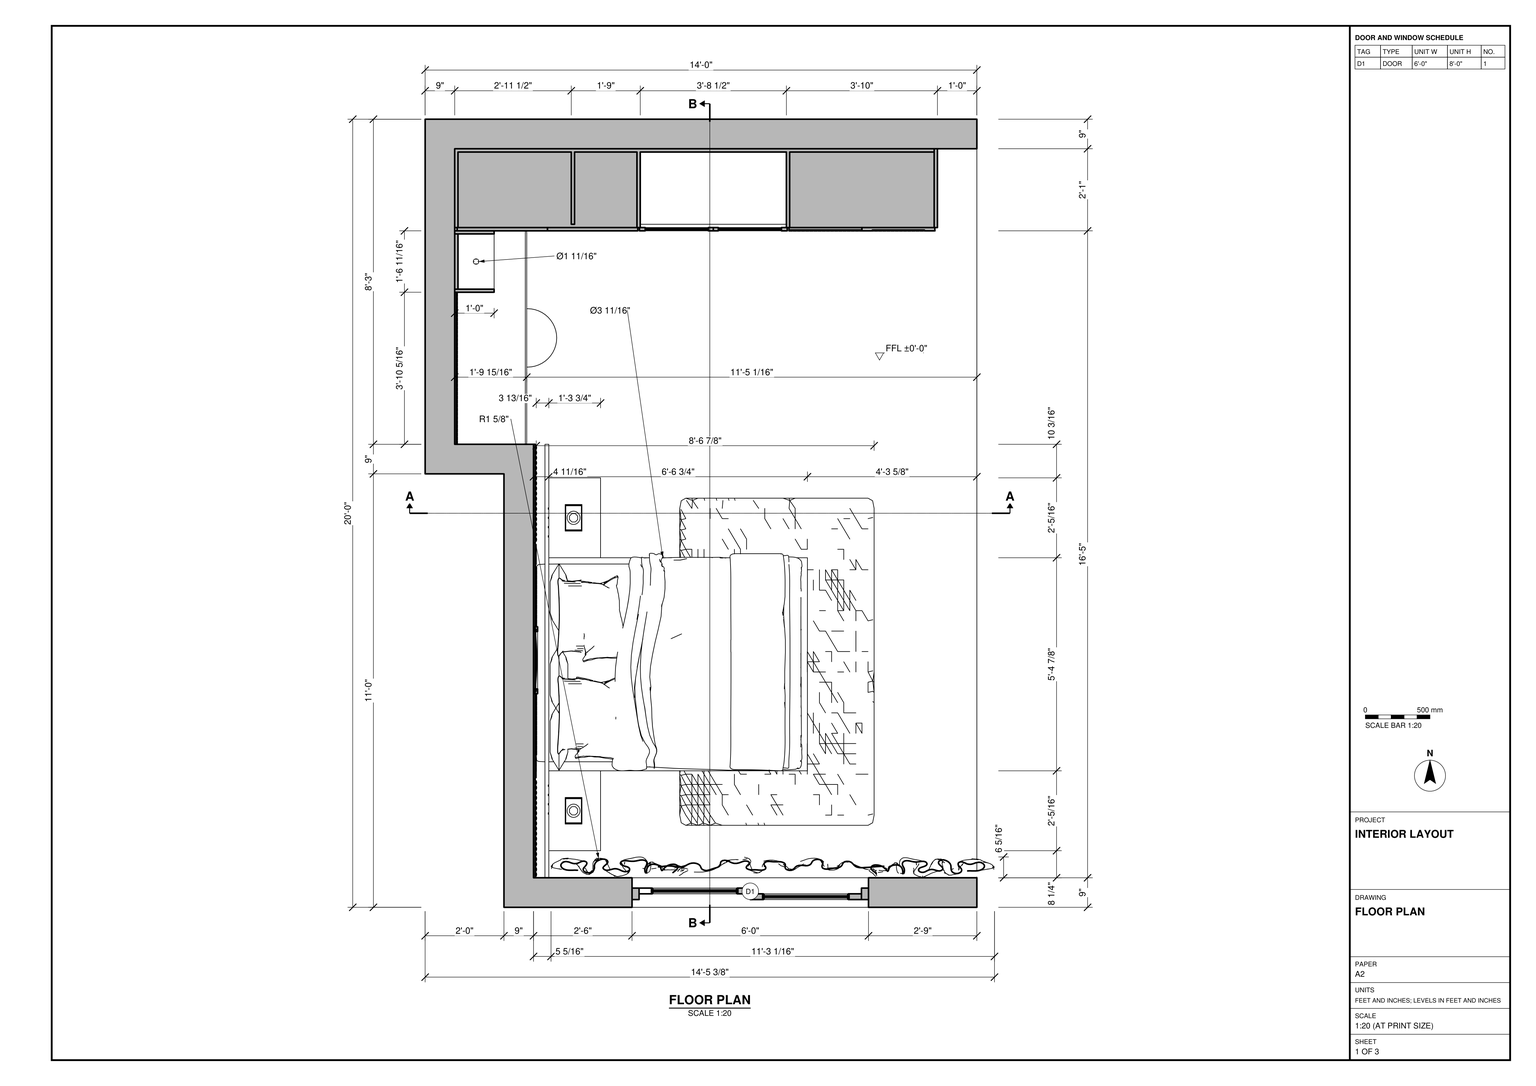
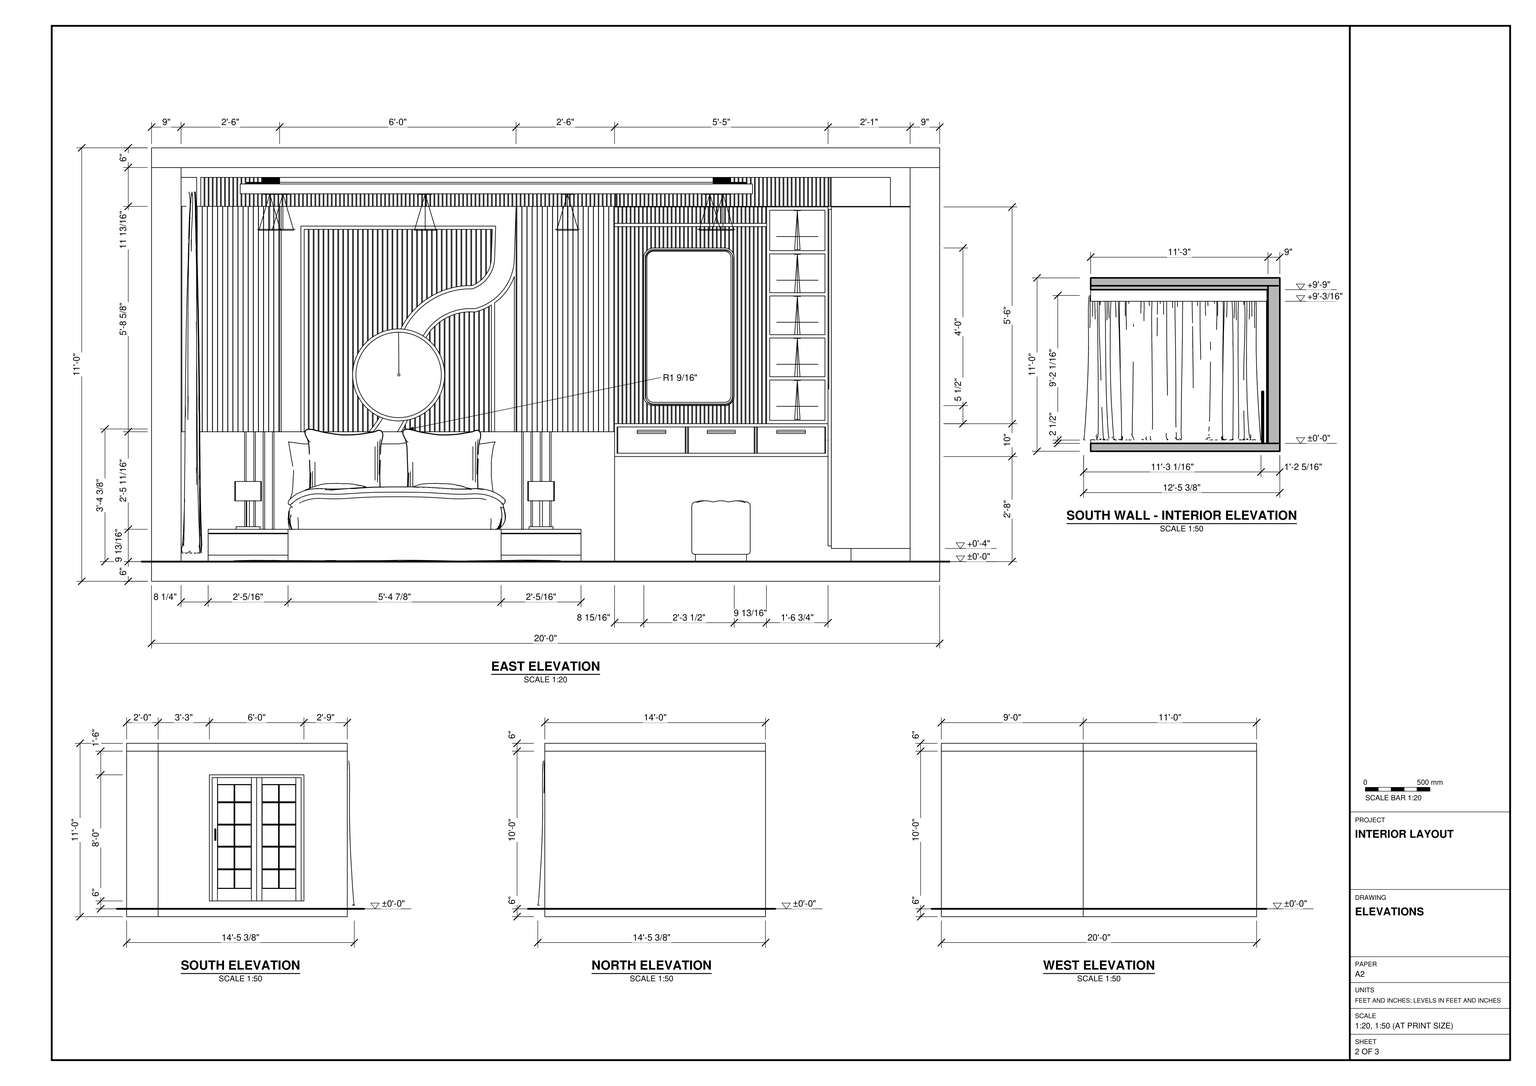
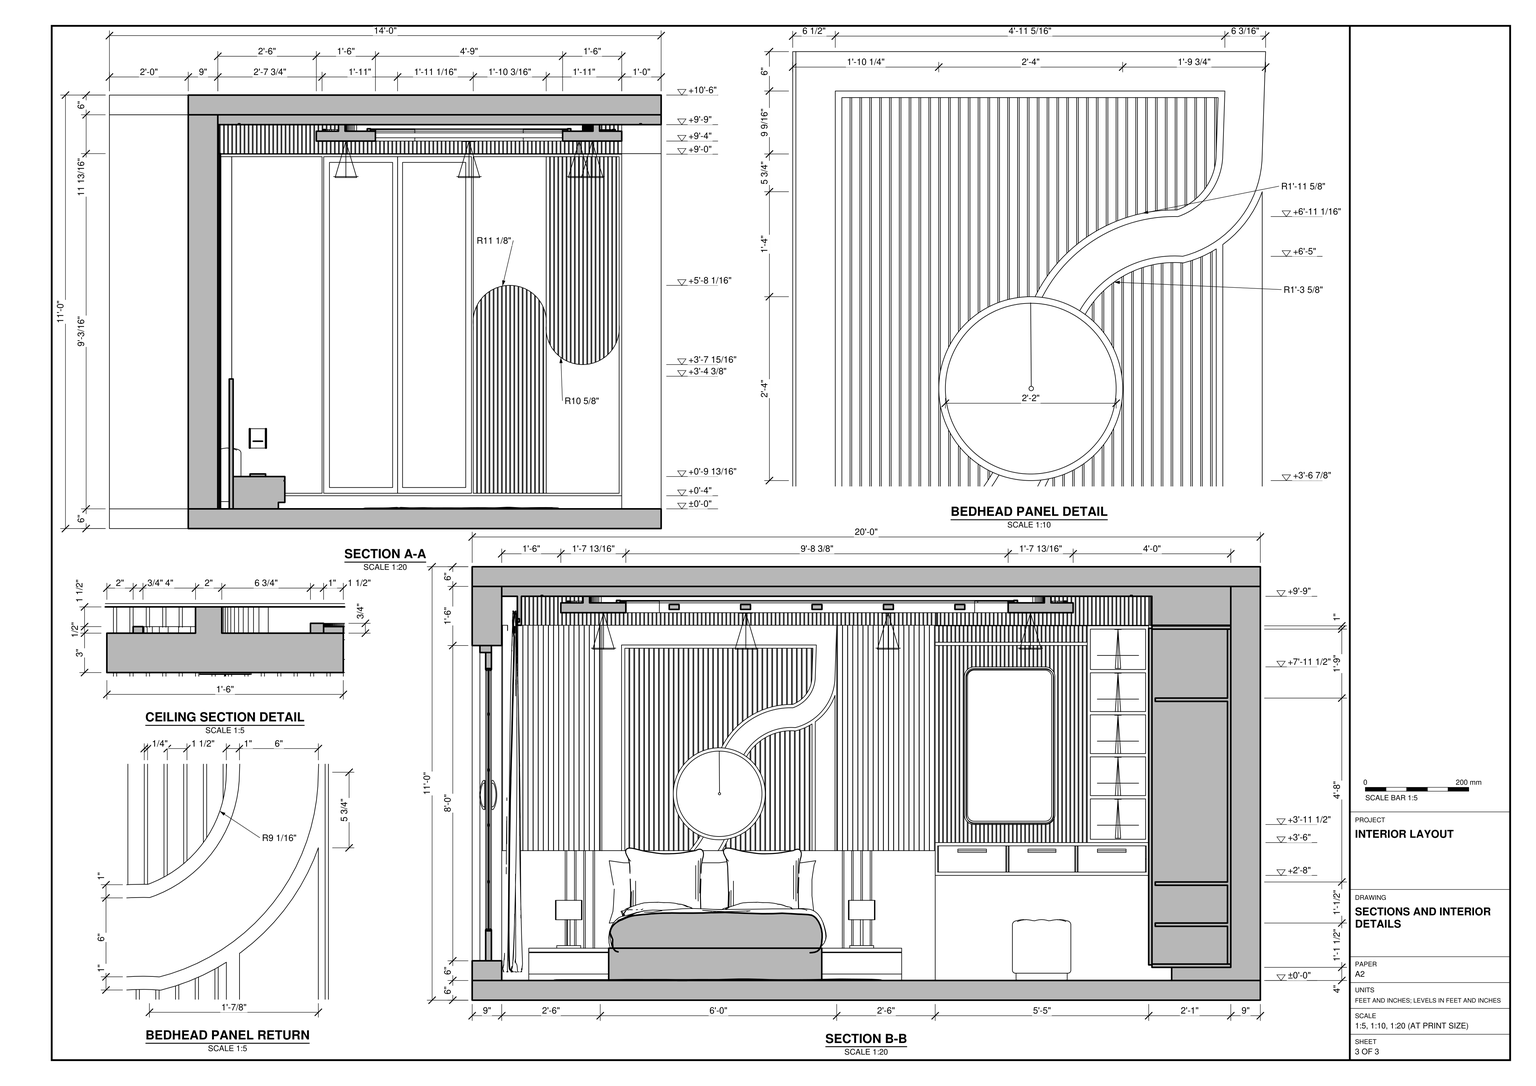
Build the bedroom interior in SketchUp from task_files/diagram_01.pdf. Work in feet and inches. The finished model measures 14'-5 3/8" east to west, 20'-0" north to south and 11'-0" high, with one finished floor level at ±0'-0". Follow the stepped west wall in plan and leave the east side open as drawn. Model the 9" walls, the floor and overhead slabs, and the glazed sliding door in the south wall. Use the sections to set out the ceiling detail above the bed and dressing area.

Place the bed with its head against the inset length of the west wall and a low bedside unit on each side. Follow the enlarged detail for the vertical ribs, circular centre and curved band of the bedhead panel. Fit the dressing counter, drawers, mirror, side shelving and stool into the wider part of the room. Continue the storage along the north wall, matching the panel divisions and curved ribbed fronts in section. Include the curtain at the south door and the rug extending beyond the foot of the bed. Decor and loose items may be any suitable library components placed as shown.

Keep the walls and slabs in separate groups or components, group each furniture or joinery piece separately, and use components for repeated parts. Save one SketchUp model as output_files/bedroom_with_a_stepped_plan_and_built_in_dressing_area.skp.

# SketchUp Ruby script. Lengths in inches.
U = 1.inch
M = Sketchup.active_model
def pt(a) = Geom::Point3d.new(a.map { |v| v * U })
def face(e, loops, mat)
  f = e.add_face(loops[0].map { |a| pt(a) })
  loops[1..].each { |l| e.add_face(l.map { |a| pt(a) }).erase! }
  f.material = f.back_material = mat if mat
  f
end
# faces: each face lists its corners as indices into pts; further lists are holes
def faces(e, pts, list, mat = nil) = list.each { |f| face(e, (f[0].is_a?(Array) ? f : [f]).map { |l| l.map { |i| pts[i] } }, mat) }
# xy, xz, yz: faces in a plane at the given z, y or x. An outline is a flat list of corners, or four numbers for a rectangle; further outlines are holes
def ring(l) = l.size == 4 ? [[l[0], l[1]], [l[2], l[1]], [l[2], l[3]], [l[0], l[3]]] : l.each_slice(2).to_a
def flat(e, list, mat, &to3) = list.each { |f| face(e, (f[0].is_a?(Array) ? f : [f]).map { |l| ring(l).map { |u, v| to3.(u, v) } }, mat) }
def xy(e, z, list, mat = nil) = flat(e, list, mat) { |x, y| [x, y, z] }
def xz(e, y, list, mat = nil) = flat(e, list, mat) { |x, z| [x, y, z] }
def yz(e, x, list, mat = nil) = flat(e, list, mat) { |y, z| [x, y, z] }
def lines(e, pts, list) = list.each { |a, b| e.add_line(pt(pts[a]), pt(pts[b])) }
# prism: a flat outline (further loops are holes) pulled along v
def prism(e, loops, v, mat = nil)
  f = face(e, loops, mat); d = Geom::Vector3d.new(v.map { |x| x * U })
  f.pushpull(f.normal.samedirection?(d) ? d.length : -d.length)
end
def box(e, o, s, mat = nil) = prism(e, [[o, [o[0] + s[0], o[1], o[2]], [o[0] + s[0], o[1] + s[1], o[2]], [o[0], o[1] + s[1], o[2]]]], [0, 0, s[2]], mat)
def at(x, y, z, deg = 0) = Geom::Transformation.translation(pt([x, y, z])) * Geom::Transformation.rotation(ORIGIN, Z_AXIS, deg.degrees)
def axes(o, x, y, z) = Geom::Transformation.new([*x, 0, *y, 0, *z, 0, *pt(o).to_a, 1])
def part(name) = M.definitions.add(name)
# library, detail: a bought-in or finely detailed component or shape, given as its bounding box
def library(name, o, s) = part(name).tap { |d| box(d.entities, o, s) }
def detail(e, o, s) = box(e.add_group.entities, o, s)
def put(e, d, t, mat = nil) = e.add_instance(d, t).tap { |i| i.material = mat if mat }
def group(e, t, mat = nil) = e.add_group.tap { |g| g.transformation = t; g.material = mat if mat }.entities
root = M.entities
M.materials.add("0993 AP 7924 MOON YEAR").color = [247, 236, 211]
M.materials.add("False ceiling Light").color = [250, 225, 158]
M.materials.add("Teddy_Skin").color = [228, 212, 199]
M.materials.add("[Color_A11]").color = [255, 247, 241]
M.materials.add("[Wood Veneer 01]2").color = [66, 44, 30]
M.materials.add("[Wood Veneer 01]3").color = [120, 70, 37]
c1 = library("Group5_1",[-7.56,-66.38,0.11],[6.33,135.04,120.95])
c2 = library("1",[0,-0.85,0],[30,0.85,108.17])
c3 = library("sliding door",[152.33,87.51,0.76],[72,5.24,96])
c4 = library("Vanity Chair",[-7.875,-7.875,0],[15.75,15.75,16.41])
c5 = library("Group\#4",[0,-1.41,0],[72,1.41,108.17])
c6 = library("Group\#11",[0,-21.9375,2],[66,21.9375,76])
c7 = library("Group\#17",[-25,0,0],[25,147,104])
c8 = library("Group\#10",[0,0,-5.36],[198,135,41.44])
c9 = library("Group\#26",[0,0,-14.11],[156,93,16.11])
c10 = part("Group155\#1")
box(c10.entities,[-9.125,-4.41,0],[1,8.82,0.25])
c11 = part("Group156\#1")
box(c11.entities,[-7.875,-4.41,0],[1,8.82,0.25])
c12 = part("Group157\#1")
box(c12.entities,[-6.625,-4.41,0],[1,8.82,0.25])
c13 = part("Group158\#1")
box(c13.entities,[-5.375,-4.41,0],[1,8.82,0.25])
c14 = part("Group159\#1")
box(c14.entities,[-4.125,-4.41,0],[1,8.82,0.25])
c15 = part("Group160\#1")
box(c15.entities,[-2.875,-4.41,0],[1,8.82,0.25])
c16 = part("Group161\#1")
box(c16.entities,[-1.625,-4.41,0],[1,8.82,0.25])
c17 = part("Group162\#1")
box(c17.entities,[-0.375,-4.41,0],[1,8.82,0.25])
c18 = part("Group163\#1")
box(c18.entities,[0.875,-4.41,0],[1,8.82,0.25])
c19 = part("Group164\#1")
box(c19.entities,[2.125,-4.41,0],[1,8.82,0.25])
c20 = part("Group165\#1")
box(c20.entities,[3.375,-4.41,0],[1,8.82,0.25])
c21 = part("Group166\#1")
box(c21.entities,[4.625,-4.41,0],[1,8.82,0.25])
c22 = part("Group167\#1")
box(c22.entities,[5.875,-4.41,0],[1,8.82,0.25])
c23 = part("Group168\#1")
box(c23.entities,[7.125,-4.41,0],[1,8.82,0.25])
c24 = part("Group169\#1")
xy(c24.entities,0,[[8.375,-4.41,9.125,4.41]])
xy(c24.entities,0.25,[[8.375,-4.41,9.125,4.41]])
yz(c24.entities,8.375,[[-4.41,0,4.41,0.25]])
c25 = part("Group153\#1")
put(c25.entities,c10,at(0,0,0))
put(c25.entities,c11,at(0,0,0))
put(c25.entities,c12,at(0,0,0))
put(c25.entities,c13,at(0,0,0))
put(c25.entities,c14,at(0,0,0))
put(c25.entities,c15,at(0,0,0))
put(c25.entities,c16,at(0,0,0))
put(c25.entities,c17,at(0,0,0))
put(c25.entities,c18,at(0,0,0))
put(c25.entities,c19,at(0,0,0))
put(c25.entities,c20,at(0,0,0))
put(c25.entities,c21,at(0,0,0))
put(c25.entities,c22,at(0,0,0))
put(c25.entities,c23,at(0,0,0))
put(c25.entities,c24,at(0,0,0))
c26 = library("Group169\#2",[-32.74,-4.41,0],[65.48,8.82,0.25])
c27 = library("Group223\#2",[-70.5,-4.41,0],[141,8.82,0.25])
c28 = library("Group337\#2",[-63.25,-4.41,0],[126.75,8.82,0.25])
g1 = group(root,at(168,0,6,90))
put(g1,c1,axes([16.56,61.01,2.42],[1,0,0],[0,1,0],[0,0,0.91]))
g2 = group(g1,at(0,0,0))
xy(g2,0,[[0,0,0,144,141,144,141,135,9,135,9,0],[231,0,231,12,213,12,213,159,132,159,132,168,240,168,240,0],[132,144,141,159]],"0993 AP 7924 MOON YEAR")
xy(g2,4,[[213,12,231,159]],"0993 AP 7924 MOON YEAR")
xy(g2,6,[[0,33,9,105]],"0993 AP 7924 MOON YEAR")
xy(g2,102,[[0,33,9,105]],"0993 AP 7924 MOON YEAR")
xy(g2,120,[[0,0,9,0,9,135,141,135,141,159,231,159,231,0,240,0,240,168,132,168,132,144,0,144]],"0993 AP 7924 MOON YEAR")
xz(g2,0,[[0,0,9,120],[231,0,240,120]],"0993 AP 7924 MOON YEAR")
xz(g2,12,[[213,0,231,4]],"0993 AP 7924 MOON YEAR")
xz(g2,33,[[0,6,9,102]],"0993 AP 7924 MOON YEAR")
xz(g2,105,[[0,6,9,102]],"0993 AP 7924 MOON YEAR")
xz(g2,135,[[9,0,141,120]],"0993 AP 7924 MOON YEAR")
xz(g2,144,[[0,0,132,120]],"0993 AP 7924 MOON YEAR")
xz(g2,159,[[141,0,213,0,213,4,231,4,231,120,141,120]],"0993 AP 7924 MOON YEAR")
xz(g2,168,[[132,0,240,120]],"0993 AP 7924 MOON YEAR")
yz(g2,0,[[[0,0,144,120],[33,6,105,102]]],"0993 AP 7924 MOON YEAR")
yz(g2,9,[[[0,0,135,120],[33,6,105,102]]],"0993 AP 7924 MOON YEAR")
yz(g2,132,[[144,0,168,120]],"0993 AP 7924 MOON YEAR")
yz(g2,141,[[135,0,159,120]],"0993 AP 7924 MOON YEAR")
yz(g2,213,[[12,0,159,4]],"0993 AP 7924 MOON YEAR")
yz(g2,231,[[0,0,0,120,159,120,159,4,12,4,12,0]],"0993 AP 7924 MOON YEAR")
yz(g2,240,[[0,0,168,120]],"0993 AP 7924 MOON YEAR")
# 2 loose lines left out
put(g2,c2,at(9,135,0),"Teddy_Skin")
put(g2,c2,at(111,135,0),"Teddy_Skin")
put(g2,c3,at(-85.25,257.33,5.24,-90))
put(g2,c4,axes([173.4,136.84,0],[1.13,0,0],[0,1.13,0],[0,0,1.13]))
put(g2,c5,at(39,135,0))
put(g2,c6,axes([141,159,30],[0.98485,0,0],[0,1,0],[0,0,1]),"[Color_A11]")
put(g2,c7,at(231,12,4),"[Wood Veneer 01]3")
put(g1,c8,axes([0,0,0],[1.21212,0,0],[0,1.24444,0],[0,0,1.12]))
g3 = group(g1,at(0,0,120))
xy(g3,0,[[0,0,0,144,132,144,132,168,240,168,240,0,231,0,231,159,141,159,141,135,9,135,9,0],[9,0,9,135,141,135,141,159,231,159,231,0]])
xy(g3,6,[[0,0,240,0,240,168,132,168,132,144,0,144]])
xz(g3,0,[[0,0,240,6]])
xz(g3,144,[[0,0,132,6]])
xz(g3,168,[[132,0,240,6]])
yz(g3,0,[[0,0,144,6]])
yz(g3,132,[[144,0,168,6]])
yz(g3,240,[[0,0,168,6]])
g4 = group(g3,at(9,0,0))
xy(g4,-11.83,[[4.75,0,4.75,134.75,5,135,6,135,6,0],[216,0,216,12,197.97,12,197.97,153,132.5,153,132.5,134.75,6,134.75,6,135,132,135,132,159,222,159,222,0]])
xy(g4,-10.83,[[4.75,1,5.375,126]])
xy(g4,-9.83,[[4.75,1,5.375,126]])
xy(g4,-3,[[0,0,0,135,5,135,4.75,134.75,4.75,0],[[6,0,6,134.75,132.5,134.75,132.5,153,197.97,153,197.97,12,216,12,216,0],[12,6,191.97,6,191.97,147,138.5,147,138.5,128.75,12,128.75]],[12.5,6.5,12.5,128.25,139,128.25,139,146.5,191.47,146.5,191.47,6.5]])
xy(g4,-2.75,[[[12,6,12,128.75,138.5,128.75,138.5,147,191.97,147,191.97,6],[12.5,6.5,191.47,6.5,191.47,146.5,139,146.5,139,128.25,12.5,128.25]]])
xy(g4,0,[[0,0,222,0,222,159,132,159,132,135,0,135]])
xz(g4,0,[[4.75,-11.83,6,-11.83,6,-3,216,-3,216,-11.83,222,-11.83,222,0,0,0,0,-3,4.75,-3]])
xz(g4,1,[[4.75,-10.83,5.375,-9.83]])
xz(g4,6,[[12,-3,191.97,-2.75]])
xz(g4,6.5,[[12.5,-3,191.47,-2.75]])
xz(g4,12,[[197.97,-11.83,216,-3]])
xz(g4,126,[[4.75,-10.83,5.375,-9.83]])
xz(g4,128.25,[[12.5,-3,139,-2.75]])
xz(g4,128.75,[[12,-3,138.5,-2.75]])
xz(g4,134.75,[[6,-11.83,132.5,-3]])
xz(g4,135,[[5,-11.83,5,-3,0,-3,0,0,132,0,132,-11.83]])
xz(g4,146.5,[[139,-3,191.47,-2.75]])
xz(g4,147,[[138.5,-3,191.97,-2.75]])
xz(g4,153,[[132.5,-11.83,197.97,-3]])
xz(g4,159,[[132,-11.83,222,0]])
yz(g4,0,[[0,-3,9,0],[9,-3,135,0]])
yz(g4,4.75,[[0,-11.83,0,-3,9,-3,9,-9.83,1,-9.83,1,-10.83,9,-10.83,9,-11.83],[9,-11.83,9,-10.83,126,-10.83,126,-9.83,9,-9.83,9,-3,134.75,-3,134.75,-11.83]])
yz(g4,5.375,[[1,-10.83,126,-9.83]])
yz(g4,6,[[0,-11.83,9,-3],[9,-11.83,134.75,-3]])
yz(g4,12,[[6,-3,9,-2.75],[9,-3,128.75,-2.75]])
yz(g4,12.5,[[6.5,-3,9,-2.75],[9,-3,128.25,-2.75]])
yz(g4,132,[[135,-11.83,159,0]])
yz(g4,132.5,[[134.75,-11.83,153,-3]])
yz(g4,138.5,[[128.75,-3,147,-2.75]])
yz(g4,139,[[128.25,-3,146.5,-2.75]])
yz(g4,191.47,[[6.5,-3,146.5,-2.75]])
yz(g4,191.97,[[6,-3,147,-2.75]])
yz(g4,197.97,[[12,-11.83,153,-3]])
yz(g4,216,[[0,-11.83,9,-3],[9,-11.83,12,-3]])
yz(g4,222,[[0,-11.83,9,0],[9,-11.83,159,0]])
p = [[4.75,134.75,-3],[5,135,-3],[5,135,-11.83],[4.75,134.75,-11.83]]
faces(g4,p,[[0,1,2,3]])
put(g4,c9,at(18,12,-5))
g5 = group(g4,at(6,12,-11.83))
p = [[0,122.75,8.83],[0,122.75,0],[126.5,122.75,0],[126.5,141,0],[191.97,141,0],[126.5,122.75,8.83],
  [126.5,141,8.83],[191.97,141,8.83],[191.97,0,0],[191.97,0,8.83]]
lines(g5,p,[[0,1],[2,3],[3,4],[0,5],[1,2],[5,6],[6,3],[6,7],[8,9],[4,7],[4,8],[7,9],
  [5,2]])
put(g5,c25,axes([126.5,131.875,4.41],[0,1,0],[0,0,1],[1,0,0]),"[Wood Veneer 01]2")
put(g5,c26,axes([159.11,141,4.41],[0.99618,0,0],[0,0,1],[0,-1,0]),"[Wood Veneer 01]2")
put(g5,c27,axes([191.97,70.5,4.41],[0,-1,0],[0,0,1],[-1,0,0]),"[Wood Veneer 01]2")
put(g5,c28,axes([63.25,122.75,4.41],[1,0,0],[0,0,1],[0,-1,0]),"[Wood Veneer 01]2")
g6 = group(g4,at(12,6,-2.75),"False ceiling Light")
prism(g6,[[[0,3,-0.25],[0,122.75,-0.25],[126.5,122.75,-0.25],[126.5,141,-0.25],[179.97,141,-0.25],[179.97,0,-0.25],[0,0,-0.25]],[[0.5,122.25,-0.25],[0.5,3,-0.25],[0.5,0.5,-0.25],[179.47,0.5,-0.25],[179.47,140.5,-0.25],[127,140.5,-0.25],[127,122.25,-0.25]]],[0,0,0.25])
g7 = group(g4,at(5.375,0,-10.83),"False ceiling Light")
box(g7,[-0.625,1,0],[0.625,125,1])
